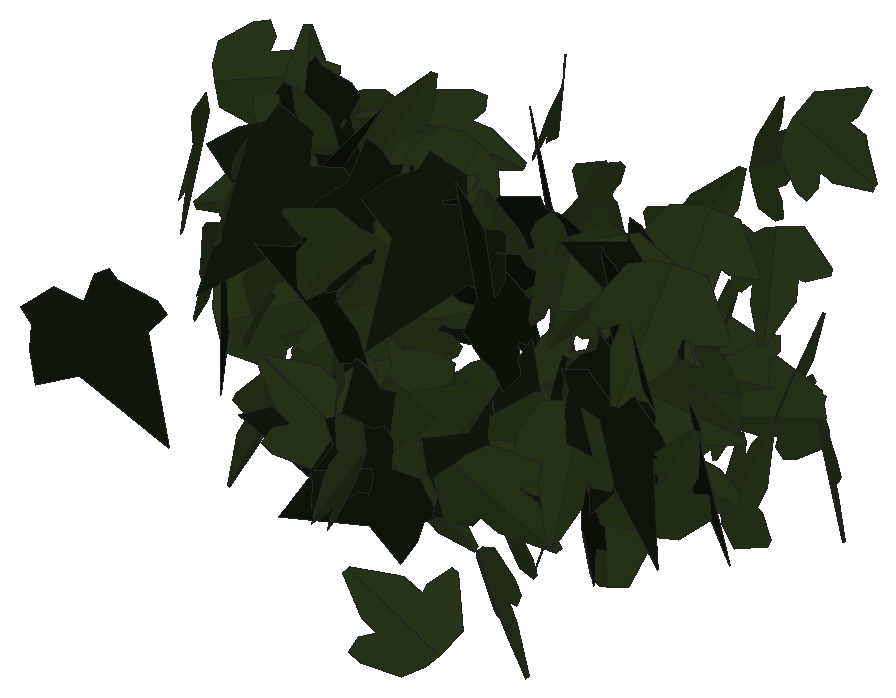
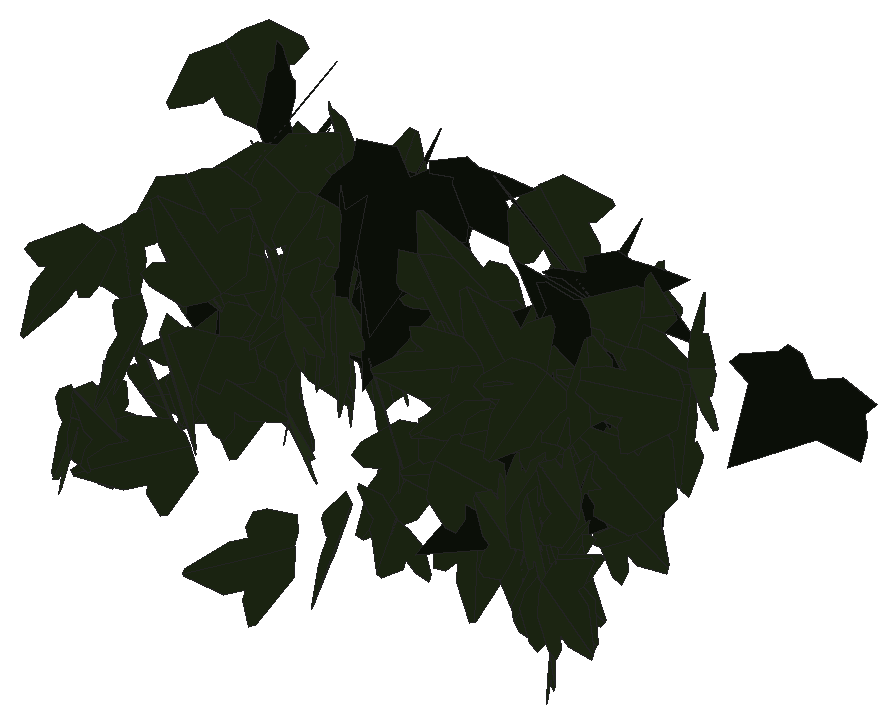
# SketchUp Ruby script. Lengths in inches.
U = 1.inch
M = Sketchup.active_model
def pt(a) = Geom::Point3d.new(a.map { |v| v * U })
def face(e, loops, mat)
  f = e.add_face(loops[0].map { |a| pt(a) })
  loops[1..].each { |l| e.add_face(l.map { |a| pt(a) }).erase! }
  f.material = f.back_material = mat if mat
  f
end
# faces: each face lists its corners as indices into pts; further lists are holes
def faces(e, pts, list, mat = nil) = list.each { |f| face(e, (f[0].is_a?(Array) ? f : [f]).map { |l| l.map { |i| pts[i] } }, mat) }
# xy, xz, yz: faces in a plane at the given z, y or x. An outline is a flat list of corners, or four numbers for a rectangle; further outlines are holes
def ring(l) = l.size == 4 ? [[l[0], l[1]], [l[2], l[1]], [l[2], l[3]], [l[0], l[3]]] : l.each_slice(2).to_a
def flat(e, list, mat, &to3) = list.each { |f| face(e, (f[0].is_a?(Array) ? f : [f]).map { |l| ring(l).map { |u, v| to3.(u, v) } }, mat) }
def xy(e, z, list, mat = nil) = flat(e, list, mat) { |x, y| [x, y, z] }
def xz(e, y, list, mat = nil) = flat(e, list, mat) { |x, z| [x, y, z] }
def yz(e, x, list, mat = nil) = flat(e, list, mat) { |y, z| [x, y, z] }
def lines(e, pts, list) = list.each { |a, b| e.add_line(pt(pts[a]), pt(pts[b])) }
# prism: a flat outline (further loops are holes) pulled along v
def prism(e, loops, v, mat = nil)
  f = face(e, loops, mat); d = Geom::Vector3d.new(v.map { |x| x * U })
  f.pushpull(f.normal.samedirection?(d) ? d.length : -d.length)
end
def box(e, o, s, mat = nil) = prism(e, [[o, [o[0] + s[0], o[1], o[2]], [o[0] + s[0], o[1] + s[1], o[2]], [o[0], o[1] + s[1], o[2]]]], [0, 0, s[2]], mat)
def at(x, y, z, deg = 0) = Geom::Transformation.translation(pt([x, y, z])) * Geom::Transformation.rotation(ORIGIN, Z_AXIS, deg.degrees)
def axes(o, x, y, z) = Geom::Transformation.new([*x, 0, *y, 0, *z, 0, *pt(o).to_a, 1])
def part(name) = M.definitions.add(name)
# library, detail: a bought-in or finely detailed component or shape, given as its bounding box
def library(name, o, s) = part(name).tap { |d| box(d.entities, o, s) }
def detail(e, o, s) = box(e.add_group.entities, o, s)
def put(e, d, t, mat = nil) = e.add_instance(d, t).tap { |i| i.material = mat if mat }
def group(e, t, mat = nil) = e.add_group.tap { |g| g.transformation = t; g.material = mat if mat }.entities
root = M.entities
M.materials.add("efeu1").color = [18, 25, 13]
M.materials.add("efeu2").color = [43, 57, 29]
c1 = part("ivyleaf_10")
p = [[0,0.5,-0.03],[-0.0625,2.02,-0.43],[-0.19,2.01,-0.46],[-0.54,1.05,-0.29],[-0.52,0.625,-0.18],[-0.83,0.76,-0.28],
  [-1.16,0.64,-0.33],[-1.15,0.33,-0.24],[-0.77,-0.39,0.02],[-0.3,-0.51,0.16],[0.04,-0.48,0.23],[-0.02,2.01,-0.4375],
  [-0.06,2.01,-0.43],[0.04,-0.49,0.23],[0.67,-0.49,0.14],[1.38,0.36,-0.2],[1.375,0.51,-0.24],[0.81,0.65,-0.19],
  [0.62,0.59,-0.15],[0.6,1.09,-0.28],[0.5,1.23,-0.31]]
faces(c1.entities,p,[[0,1,2,3,4,5,6,7,8,9,10],[11,12,0,13,14,15,16,17,18,19,20]],"efeu2")
c2 = part("ivyleaf_9")
p = [[1.54,2.16,1.25],[1.36,2.04,1.19],[-0.21,0.99,0.68],[-0.71,1.11,0.82],[-0.85,0.86,0.67],[-0.8,0.17,0.21],
  [-0.9,-0.01,0.1],[-0.67,-0.16,-0.02],[-0.08,-0.08,-0.05],[-0.03,-0.6,-0.4],[0.65,-0.88,-0.66],[0.83,-0.6,-0.49],
  [1.29,-0.42,-0.43],[1.8125,-0.07,-0.26],[1.21,0.44,0.15]]
faces(c2.entities,p,[[0,1,2,3,4,5,6,7,8,9,10,11,12,13,14]],"efeu1")
put(root,c1,axes([516.52,137.66,156.65],[0.08442,0.01855,-0.6977],[0.67328,0.183,0.08633],[0.18389,-0.67854,0.00421]))
put(root,c1,axes([516.84,136.29,156.4],[0.26213,-0.2531,0.68432],[0.47052,-0.4971,-0.36409],[0.55764,0.53842,-0.01447]))
put(root,c1,axes([517.24,139.04,153.74],[0.1329,-0.54962,0.31428],[0.06196,-0.3083,-0.56535],[0.63009,0.14624,-0.01069]))
put(root,c2,axes([517.03,133.52,154.87],[-0.20979,-0.28706,-0.70219],[0.45244,0.53744,-0.35488],[0.60891,-0.49824,0.02177]))
put(root,c1,axes([517.36,136.1,154.6],[0.07095,-0.52051,-0.47781],[0.062,-0.47378,0.52532],[-0.70384,-0.0942,-0.00189]))
put(root,c1,axes([517.59,137.73,156.08],[0.15222,0.70501,-0.21929],[0.04502,0.21462,0.72125],[0.73695,-0.15873,0.00123]))
put(root,c1,axes([517.2,137.19,154.55],[-0.43761,-0.17389,0.55924],[0.51418,0.22014,0.4708],[-0.28037,0.67512,-0.00947]))
put(root,c1,axes([518.02,138.19,152.4],[0.05804,0.00502,0.65259],[-0.52703,0.38676,0.0439],[-0.38489,-0.52883,0.03829]))
put(root,c1,axes([517.71,138.2,154.66],[0.23347,-0.49596,0.3383],[-0.16672,0.29514,0.54774],[-0.57673,-0.28609,-0.02139]))
put(root,c1,axes([517.8,138.48,153.41],[-0.11161,-0.50792,0.38042],[-0.01849,-0.38349,-0.51745],[0.63432,-0.10055,0.05185]))
put(root,c1,axes([517.76,138.84,154.78],[0.17832,-0.6274,-0.0109],[-0.00363,0.0103,-0.65225],[0.62748,0.17836,-0.00067]))
put(root,c1,axes([518.05,138.38,154.27],[0.36729,-0.45852,-0.26908],[-0.18085,0.19979,-0.5873],[0.49994,0.40914,-0.01477]))
put(root,c2,axes([517.58,136.03,154.88],[-0.02809,-0.00164,-0.77935],[0.7183,-0.30263,-0.02525],[-0.30238,-0.71874,0.01241]))
put(root,c1,axes([518.47,137.19,156.39],[-0.28555,-0.02384,0.59598],[-0.59398,-0.04877,-0.28654],[0.05428,-0.65906,-0.00035]))
put(root,c1,axes([518,138.57,153.19],[-0.13395,0.38373,0.64136],[0.16194,-0.6212,0.40549],[0.72963,0.20832,0.02775]))
put(root,c1,axes([518.1,137.73,154.33],[-0.09057,-0.22912,0.6866],[0.04471,-0.69241,-0.22516],[0.72244,0.01413,0.10001]))
put(root,c1,axes([518.7,136.24,156.21],[-0.15275,-0.12758,0.73648],[-0.57683,-0.45793,-0.19896],[0.47534,-0.59669,-0.00477]))
put(root,c1,axes([518.51,138.4,154.45],[-0.45096,0.33204,-0.33354],[-0.27112,0.19432,0.56],[0.3847,0.52617,0.00367]))
put(root,c1,axes([518.1875,136.14,153.71],[0.11967,-0.41084,0.50869],[-0.06709,0.50669,0.42501],[-0.65042,-0.12786,0.04975]))
put(root,c1,axes([518.55,137.85,153.3],[-0.3026,-0.29674,0.48488],[-0.30813,-0.37599,-0.42239],[0.47772,-0.43047,0.03469]))
put(root,c1,axes([518.22,135.78,156.57],[-0.02282,0.31728,-0.58082],[0.00031,-0.58116,-0.31748],[-0.66183,-0.01121,0.01987]))
put(root,c1,axes([518.24,138.31,156.43],[-0.58903,-0.04948,-0.26134],[0.26069,0.01864,-0.59109],[0.05279,-0.64413,0.00297]))
put(root,c1,axes([518.04,135.8,154.13],[0.14434,0.05661,-0.72448],[0.61876,0.37775,0.15279],[0.38106,-0.63483,0.02632]))
put(root,c2,axes([517.97,137.36,156.91],[-0.06775,-0.1757,-0.75335],[0.72116,0.25927,-0.12532],[0.27988,-0.71057,0.14055]))
put(root,c1,axes([518.41,137.14,152.375],[0.52897,-0.38562,0.0331],[-0.02481,0.02216,0.6546],[-0.38625,-0.52954,0.00329]))
put(root,c1,axes([518.53,138.61,154.04],[0.27358,-0.48885,0.32679],[-0.16228,0.28366,0.56019],[-0.56518,-0.31808,-0.00266]))
put(root,c1,axes([518.44,135.9,155.28],[-0.04464,-0.34452,-0.63146],[0.19241,0.6039,-0.34309],[0.69312,-0.18983,0.05458]))
put(root,c2,axes([518.8,137.59,152.92],[0.24441,-0.54795,0.47861],[-0.15917,0.4524,0.59921],[-0.70992,-0.29008,0.03043]))
put(root,c1,axes([518.29,138.22,155.9],[-0.25929,-0.05729,-0.58922],[0.58567,0.06902,-0.26443],[0.08637,-0.64004,0.02422]))
put(root,c1,axes([518.71,135.76,153.16],[0.12292,-0.58224,0.4466],[0.08398,-0.43869,-0.59504],[0.72898,0.14871,-0.00676]))
put(root,c2,axes([518.54,136.21,155.71],[0.14157,0.74264,0.09302],[-0.0357,-0.08786,0.75579],[0.74759,-0.14482,0.01848]))
put(root,c2,axes([519.18,135.78,156.875],[-0.69635,-0.38468,0.06883],[-0.05391,-0.04474,-0.79543],[0.38705,-0.69831,0.01305]))
put(root,c2,axes([518.5,137.62,154.39],[0.0481,-0.09955,-0.7675],[0.35782,0.68471,-0.06639],[0.68624,-0.35005,0.08841]))
put(root,c1,axes([519.04,137.875,156.33],[-0.31979,-0.5378,0.23744],[0.13702,0.19467,0.62546],[-0.5717,0.34749,0.01709]))
put(root,c1,axes([519.3125,138.75,154.9375],[-0.07391,-0.39629,0.5287],[-0.03141,-0.52928,-0.40112],[0.65998,-0.06957,0.04012]))
put(root,c1,axes([519.11,138.3,155.71],[0.26272,0.57552,0.13059],[0.05607,0.11796,-0.63264],[-0.58748,0.26863,-0.00198]))
put(root,c1,axes([518.87,137.69,153.25],[-0.01304,-0.1435,0.7618],[0.63373,-0.44077,-0.07218],[0.44645,0.62147,0.12471]))
put(root,c1,axes([519.53,138.32,155.5625],[0.47779,0.29842,-0.4379],[-0.36933,-0.23529,-0.56332],[-0.38001,0.60389,-0.00309]))
put(root,c1,axes([518.96,137.7,155.18],[-0.03862,-0.03541,-0.64209],[0.63688,0.08686,-0.0431],[0.08894,-0.63736,0.0298]))
put(root,c1,axes([519.16,136.3,153.3],[0.34161,0.06767,-0.63982],[0.46894,0.46979,0.30007],[0.4405,-0.5526,0.17675]))
put(root,c1,axes([519.29,137.875,155.89],[-0.11565,-0.19552,-0.63132],[0.38475,0.5012,-0.2257],[0.53737,-0.40093,0.02573]))
put(root,c2,axes([519.16,135.99,155.74],[0.24598,0.41255,-0.61579],[0.25969,0.55972,0.47872],[0.69423,-0.35555,0.03911]))
put(root,c1,axes([519.32,136.06,153.78],[-0.2872,-0.09268,-0.7207],[0.70923,0.13285,-0.29971],[0.15809,-0.76435,0.0353]))
put(root,c2,axes([519.875,137.35,155.94],[-0.58366,0.21153,-0.47041],[0.44336,-0.15725,-0.62081],[-0.26357,-0.73295,-0.00257]))
put(root,c1,axes([519.43,138.52,156.48],[-0.19774,-0.06266,-0.62741],[0.62923,0.02262,-0.20057],[0.04049,-0.65745,0.0529]))
put(root,c1,axes([519.68,136.6875,155.64],[0.06658,-0.1085,0.70684],[0.36704,-0.60407,-0.1273],[0.61374,0.37303,-0.00054]))
put(root,c1,axes([519.51,136.1875,154.49],[-0.35842,-0.10856,0.59966],[0.56685,0.196,0.37429],[-0.22372,0.67055,-0.01232]))
put(root,c2,axes([519.91,135.54,155.09],[0.43515,-0.67144,-0.05441],[0.03256,-0.04374,0.80011],[-0.67285,-0.43636,0.00352]))
put(root,c1,axes([519.64,137.73,154.38],[-0.21432,-0.06195,-0.61418],[0.61712,-0.03684,-0.21164],[-0.01456,-0.64945,0.07059]))
put(root,c1,axes([520,137.13,153.86],[-0.57759,-0.19976,0.23763],[0.22355,0.08061,0.61115],[-0.21539,0.61934,-0.0029]))
put(root,c1,axes([520.35,134.99,153.43],[0.29512,0.54373,0.45632],[-0.21583,-0.40205,0.61866],[0.67623,-0.36562,-0.00169]))
put(root,c1,axes([519.92,135.4,154.12],[0.51411,-0.29877,0.32403],[0.28277,-0.15829,-0.5946],[0.33808,0.58673,0.00459]))
put(root,c1,axes([520.3,136.95,152.86],[-0.2941,-0.58216,-0.07966],[0.03664,0.07074,-0.65223],[0.58644,-0.29637,0.00079]))
put(root,c2,axes([520.9,134.875,153.39],[-0.48027,0.24968,0.55378],[-0.49143,0.25528,-0.5413],[-0.35709,-0.68714,0.00012]))
put(root,c2,axes([520.87,135.13,156.9],[-0.52261,0.44761,0.35493],[-0.2683,0.23238,-0.68809],[-0.50433,-0.58745,-0.00175]))
put(root,c1,axes([520.0625,137.28,154.9375],[0.74532,-0.09526,-0.21151],[0.2108,-0.01895,0.75135],[-0.09682,-0.77452,0.00763]))
put(root,c1,axes([520.53,136.51,155.81],[-0.62419,-0.40897,0.1618],[-0.13292,-0.09237,-0.74623],[0.41925,-0.63817,0.00432]))
put(root,c1,axes([520.66,139.65,154.01],[-0.1897,0.3296,0.51373],[-0.2718,0.43607,-0.38014],[-0.54651,-0.33128,0.01074]))
put(root,c1,axes([520.875,134.65,156.85],[-0.49933,-0.27935,0.38802],[-0.33346,-0.1986,-0.57209],[0.34264,-0.60037,0.0087]))
put(root,c1,axes([520.89,139.38,157.13],[0.18478,-0.5391,-0.35135],[-0.10072,0.33681,-0.56977],[0.63555,0.21012,0.01185]))
put(root,c1,axes([520.9,137.25,156.94],[0.6885,-0.08443,-0.21605],[-0.21434,0.02718,-0.69366],[0.08869,0.72109,0.00085]))
put(root,c2,axes([521.5,134.77,153.24],[0.04347,0.05773,-0.77306],[-0.61277,-0.4717,-0.06968],[-0.47483,0.61401,0.01915]))
put(root,c1,axes([521.08,137.84,152.99],[0.55338,-0.06363,0.36928],[0.36519,-0.05604,-0.55691],[0.08399,0.66292,-0.01163]))
put(root,c1,axes([521.09,135.91,155.84],[0.72629,0.09781,-0.40417],[0.39227,0.10884,0.73124],[0.13802,-0.82402,0.04861]))
put(root,c1,axes([521.36,136.89,153.66],[-0.56554,-0.28096,-0.38375],[0.33523,0.18747,-0.63128],[0.33738,-0.65724,-0.01602]))
put(root,c1,axes([521.37,135.41,154.26],[-0.23605,0.00003,-0.6743],[0.65072,-0.18727,-0.2278],[-0.17676,-0.68945,0.06184]))
put(root,c1,axes([521.55,135.24,152.98],[-0.33699,0.11442,-0.62069],[0.57848,-0.2254,-0.35563],[-0.25241,-0.66934,0.01365]))
put(root,c2,axes([522.2,135.57,157.29],[-0.69816,-0.41465,-0.00161],[0.00598,-0.00692,-0.81196],[0.41461,-0.69813,0.00901]))
put(root,c1,axes([521.92,133.39,154.11],[0.03485,-0.01536,0.72305],[0.36603,-0.62395,-0.03089],[0.62375,0.36701,-0.02227]))
put(root,c1,axes([521.75,137.1,153.68],[0.20663,-0.22156,-0.6991],[0.43122,-0.55079,0.30201],[-0.5932,-0.47756,-0.02398]))
put(root,c2,axes([522.32,135.71,156.4],[0.64103,0.44977,-0.1962],[-0.15853,-0.11566,-0.78307],[-0.46439,0.66033,-0.00352]))
put(root,c2,axes([522.43,135.91,157.28],[0.50318,0.52901,-0.2124],[-0.15922,-0.14161,-0.7299],[-0.54737,0.5275,0.01707]))
put(root,c1,axes([522.26,139.13,152.74],[0.03678,0.0363,-0.75049],[0.38052,0.647,0.04994],[0.64789,-0.38207,0.01327]))
put(root,c2,axes([522.84,136.99,156.1],[0.15144,-0.35778,0.66963],[-0.15104,0.65497,0.38411],[-0.74404,-0.20578,0.05832]))
put(root,c1,axes([522.51,138.36,156.29],[0.23105,-0.48007,0.40784],[0.19939,-0.35633,-0.5324],[0.59753,0.30454,0.01996]))
put(root,c1,axes([522.9,135.95,156.36],[-0.73199,-0.18456,-0.21761],[-0.20633,-0.07149,0.75468],[-0.19709,0.7603,0.01813]))
put(root,c1,axes([523.04,134.875,154.69],[-0.34894,-0.40693,0.41414],[-0.25942,-0.32299,-0.53595],[0.51943,-0.43468,0.01053]))
put(root,c1,axes([522.6,138.22,154.42],[0.38823,-0.37303,0.48077],[0.33256,-0.34752,-0.53819],[0.5096,0.51097,-0.01505]))
put(root,c1,axes([522.71,138.02,156.65],[0.04849,-0.19011,0.65797],[0.28521,-0.5941,-0.19267],[0.62267,0.28693,0.03702]))
put(root,c2,axes([523.24,135.47,155.76],[-0.03449,-0.70959,0.40892],[0.05888,0.40607,0.70961],[-0.81686,0.05923,0.03389]))
put(root,c1,axes([523.07,137.28,157.04],[-0.11145,-0.54646,-0.44472],[0.08938,0.43564,-0.55771],[0.69886,-0.14287,0.00041]))
put(root,c1,axes([523.11,136.95,156.01],[-0.03736,0.23931,0.73813],[-0.09556,0.73194,-0.24214],[-0.77005,-0.10244,-0.00576]))
put(root,c1,axes([523.08,136.98,154.58],[-0.47648,0.28019,0.39589],[0.32503,-0.22744,0.55217],[0.35999,0.57622,0.02544]))
put(root,c1,axes([523.03,135.32,153.99],[0.08012,-0.0853,0.72007],[0.59595,-0.40495,-0.11428],[0.41307,0.60078,0.02521]))
put(root,c1,axes([523.72,140.55,156.43],[-0.10848,0.19287,0.66736],[-0.32771,0.58136,-0.22129],[-0.61252,-0.3452,0.0002]))
put(root,c1,axes([523.76,132.66,152.26],[0.29633,0.50117,0.46093],[-0.23061,-0.39911,0.58221],[0.64066,-0.37547,-0.00363]))
put(root,c2,axes([523.67,134.57,153.7],[-0.51666,-0.2467,0.52778],[0.47758,0.22467,0.57253],[-0.33367,0.70357,0.00224]))
put(root,c1,axes([524.01,135.44,157.34],[0.50507,-0.49047,-0.24955],[-0.16263,0.19055,-0.70369],[0.52573,0.53015,0.02206]))
put(root,c1,axes([523.37,136.07,154.76],[0.29393,-0.25205,-0.63911],[0.60777,-0.22872,0.36972],[-0.32033,-0.66524,0.11504]))
put(root,c1,axes([524.35,136.09,154.38],[-0.43117,-0.12625,0.49892],[-0.46464,-0.18438,-0.4482],[0.22129,-0.63312,0.03104]))
put(root,c1,axes([523.7,134.67,153.15],[-0.54359,0.03892,0.52665],[0.5061,-0.17745,0.53549],[0.15081,0.73578,0.10129]))
put(root,c1,axes([524.22,137.82,154.32],[-0.08811,-0.42013,0.50884],[-0.06046,-0.50606,-0.4283],[0.65709,-0.1029,0.02882]))
put(root,c1,axes([524.26,136.43,156.97],[-0.16269,-0.56482,0.49986],[-0.0691,-0.49805,-0.58526],[0.75107,-0.16817,0.05443]))
put(root,c1,axes([524.09,138.39,156.33],[-0.33154,-0.50986,0.30712],[0.15799,0.26356,0.60809],[-0.57386,0.36713,-0.01003]))
put(root,c1,axes([523.92,134.62,154.59],[0.03073,-0.04265,0.68193],[0.42766,0.53357,0.0141],[-0.53287,0.42576,0.05063]))
put(root,c1,axes([524.58,134.73,153.93],[0.30094,-0.59491,-0.43946],[-0.19326,0.39472,-0.66668],[0.71393,0.35762,0.00478]))
put(root,c1,axes([524.2,138.14,154.92],[0.47979,0.46364,0.20836],[0.14397,0.15084,-0.66715],[-0.4875,0.50085,0.00804]))
put(root,c1,axes([524.42,138.76,155.02],[0.43726,-0.63537,0.05467],[0.03548,-0.04195,-0.77128],[0.63673,0.43866,0.00544]))
put(root,c1,axes([524.15,139.25,153.77],[-0.17485,-0.11704,-0.63146],[0.58555,0.23973,-0.20657],[0.26376,-0.60979,0.03999]))
put(root,c1,axes([524.25,133.35,154.7],[-0.54054,-0.10909,-0.53123],[0.52005,0.10845,-0.55143],[0.1538,-0.75009,-0.00247]))
put(root,c1,axes([524.43,136.17,157.03],[0.49392,0.50186,0.11537],[0.0801,0.08304,-0.70415],[-0.50869,0.50037,0.00114]))
put(root,c1,axes([524.78,135.7,152.57],[0.67429,-0.18321,0.26968],[-0.26169,0.06536,0.69872],[-0.19445,-0.72327,-0.00517]))
put(root,c1,axes([524.74,136.15,155.63],[0.50288,-0.50567,0.00594],[0.00423,-0.00417,-0.71316],[0.50569,0.5029,0.00006]))
put(root,c1,axes([524.65,140.47,157.35],[0.08763,0.51977,0.47683],[0.07003,0.47171,-0.52706],[-0.70187,0.11196,0.00694]))
put(root,c2,axes([524.69,134.97,154.8],[-0.43797,0.61334,0.34607],[0.19669,-0.28479,0.75365],[0.67621,0.48009,0.00493]))
put(root,c2,axes([525.03,134.86,154.19],[0.30304,-0.1444,-0.69135],[-0.63562,0.27223,-0.33547],[0.30792,0.70406,-0.01209]))
put(root,c1,axes([525.06,134.38,155.45],[0.03696,-0.13669,-0.67879],[-0.16588,0.65822,-0.14158],[0.67225,0.16993,0.00239]))
put(root,c1,axes([524.9,137.62,157.07],[0.58531,0.32787,-0.18661],[-0.17076,-0.07689,-0.6707],[-0.33639,0.60951,0.01577]))
put(root,c2,axes([525.08,136.49,156.59],[0.21792,-0.72711,-0.12893],[0.03831,-0.12311,0.75907],[-0.73746,-0.22126,0.00133]))
put(root,c1,axes([525.55,139.15,153.63],[-0.07729,-0.06632,0.66836],[-0.56175,-0.36239,-0.10092],[0.36815,-0.56688,-0.01368]))
put(root,c1,axes([525.07,136.32,154.02],[-0.27144,-0.47357,-0.53168],[0.25202,0.46826,-0.54575],[0.66591,-0.37026,-0.01018]))
put(root,c1,axes([525.23,139.18,153.71],[0.26184,-0.48451,0.38681],[-0.15337,0.35622,0.55002],[-0.60071,-0.30214,0.02818]))
put(root,c1,axes([524.73,136.9375,153.61],[-0.27538,-0.01575,-0.69148],[0.69155,-0.01937,-0.27497],[-0.01217,-0.74405,0.0218]))
put(root,c1,axes([525.47,138.6,156.52],[0.24273,0.60528,-0.1459],[-0.06762,-0.13004,-0.65198],[-0.61893,0.25158,0.01401]))
put(root,c2,axes([525.06,135.36,157.14],[0.14789,-0.08299,-0.76379],[0.76517,-0.05412,0.15403],[-0.06917,-0.77609,0.07094]))
put(root,c2,axes([525.39,135.32,155.49],[0.00331,-0.62618,0.51013],[-0.0092,-0.51013,-0.62612],[0.80762,-0.00324,-0.00922]))
put(root,c1,axes([525.35,132.31,153.98],[-0.43835,0.37906,-0.48542],[0.36217,-0.32326,-0.57949],[-0.49815,-0.56858,0.00585]))
put(root,c1,axes([525.55,133.83,155.66],[0.80205,-0.163,0.05092],[0.05065,-0.00642,-0.81843],[0.16308,0.80363,0.00378]))
put(root,c1,axes([526.16,136.54,155.38],[0.23961,-0.16729,-0.63413],[-0.52641,0.3536,-0.29219],[0.39115,0.57836,-0.00478]))
put(root,c1,axes([525.34,135.97,155.22],[0.03887,0.0017,0.76415],[0.73047,0.22458,-0.03766],[-0.22437,0.73144,0.00979]))
put(root,c1,axes([525.78,135.3,153.83],[-0.47609,-0.56331,0.27317],[0.17669,0.20834,0.73755],[-0.6006,0.50782,0.00044]))
put(root,c2,axes([525.57,134.73,155.75],[0.33905,-0.78076,0.06942],[0.03935,-0.05858,-0.85111],[0.78286,0.34108,0.01272]))
put(root,c1,axes([525.83,137.27,153.14],[0.57371,-0.41831,-0.27874],[0.2438,-0.13834,0.7094],[-0.43959,-0.62266,0.02966]))
put(root,c2,axes([525.67,136.35,154.73],[0.02869,0.00619,-0.79542],[0.79264,-0.06702,0.02807],[-0.06676,-0.79311,-0.00858]))
put(root,c1,axes([526.22,135.07,157.64],[0.50588,0.59729,-0.32327],[-0.22226,-0.2353,-0.78257],[-0.64177,0.55232,0.0162]))
put(root,c1,axes([526.07,139.01,153.43],[-0.37327,0.48049,-0.3051],[0.1694,-0.25453,-0.60811],[-0.54338,-0.40942,0.02]))
